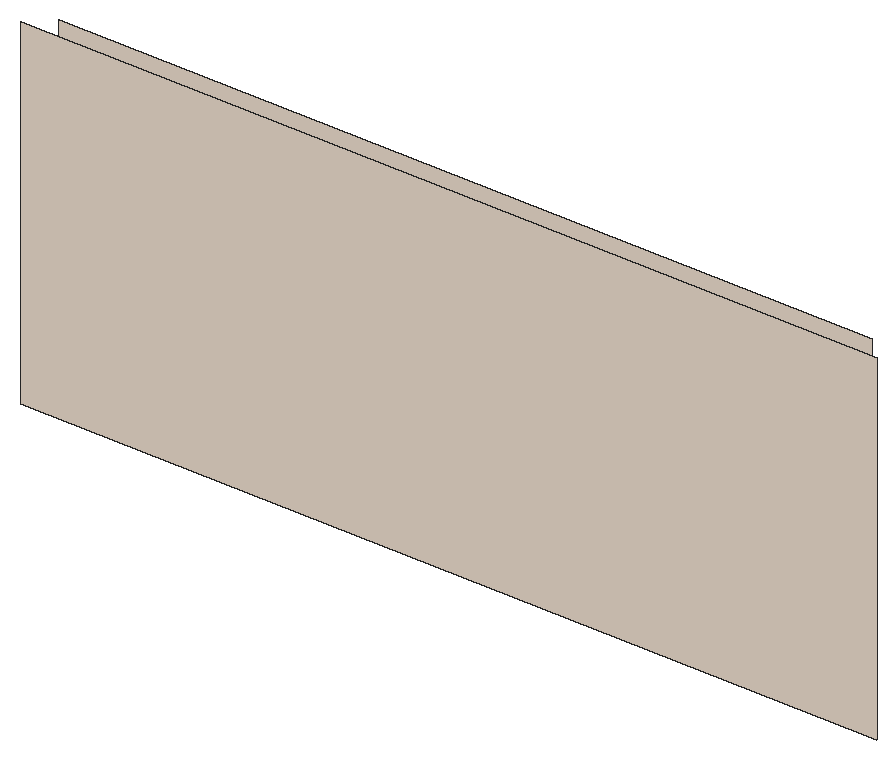
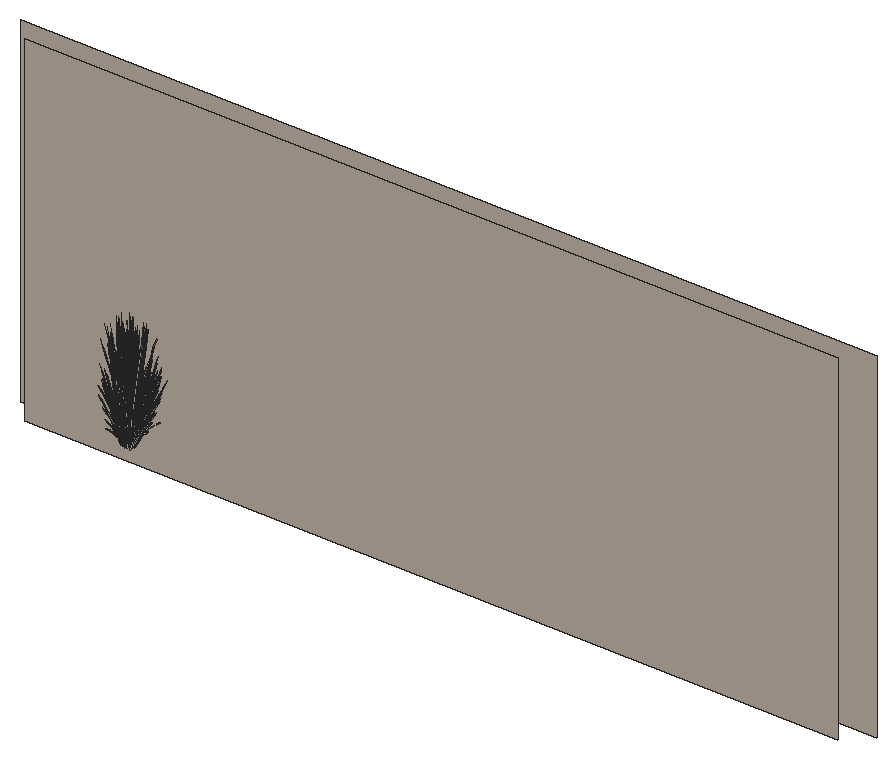
# SketchUp Ruby script. Lengths in inches.
U = 1.inch
M = Sketchup.active_model
def pt(a) = Geom::Point3d.new(a.map { |v| v * U })
def face(e, loops, mat)
  f = e.add_face(loops[0].map { |a| pt(a) })
  loops[1..].each { |l| e.add_face(l.map { |a| pt(a) }).erase! }
  f.material = f.back_material = mat if mat
  f
end
# faces: each face lists its corners as indices into pts; further lists are holes
def faces(e, pts, list, mat = nil) = list.each { |f| face(e, (f[0].is_a?(Array) ? f : [f]).map { |l| l.map { |i| pts[i] } }, mat) }
# xy, xz, yz: faces in a plane at the given z, y or x. An outline is a flat list of corners, or four numbers for a rectangle; further outlines are holes
def ring(l) = l.size == 4 ? [[l[0], l[1]], [l[2], l[1]], [l[2], l[3]], [l[0], l[3]]] : l.each_slice(2).to_a
def flat(e, list, mat, &to3) = list.each { |f| face(e, (f[0].is_a?(Array) ? f : [f]).map { |l| ring(l).map { |u, v| to3.(u, v) } }, mat) }
def xy(e, z, list, mat = nil) = flat(e, list, mat) { |x, y| [x, y, z] }
def xz(e, y, list, mat = nil) = flat(e, list, mat) { |x, z| [x, y, z] }
def yz(e, x, list, mat = nil) = flat(e, list, mat) { |y, z| [x, y, z] }
def lines(e, pts, list) = list.each { |a, b| e.add_line(pt(pts[a]), pt(pts[b])) }
# prism: a flat outline (further loops are holes) pulled along v
def prism(e, loops, v, mat = nil)
  f = face(e, loops, mat); d = Geom::Vector3d.new(v.map { |x| x * U })
  f.pushpull(f.normal.samedirection?(d) ? d.length : -d.length)
end
def box(e, o, s, mat = nil) = prism(e, [[o, [o[0] + s[0], o[1], o[2]], [o[0] + s[0], o[1] + s[1], o[2]], [o[0], o[1] + s[1], o[2]]]], [0, 0, s[2]], mat)
def at(x, y, z, deg = 0) = Geom::Transformation.translation(pt([x, y, z])) * Geom::Transformation.rotation(ORIGIN, Z_AXIS, deg.degrees)
def axes(o, x, y, z) = Geom::Transformation.new([*x, 0, *y, 0, *z, 0, *pt(o).to_a, 1])
def part(name) = M.definitions.add(name)
# library, detail: a bought-in or finely detailed component or shape, given as its bounding box
def library(name, o, s) = part(name).tap { |d| box(d.entities, o, s) }
def detail(e, o, s) = box(e.add_group.entities, o, s)
def put(e, d, t, mat = nil) = e.add_instance(d, t).tap { |i| i.material = mat if mat }
def group(e, t, mat = nil) = e.add_group.tap { |g| g.transformation = t; g.material = mat if mat }.entities
root = M.entities
M.materials.add("C01_Vanilla_Cream").color = [244, 228, 212]
M.materials.add("LightPink_Translucent").color = [144, 107, 117]
M.materials["LightPink_Translucent"].alpha = 0.75
c1 = part("blade")
p = [[2.15,0.21,22],[0,0.17,0],[0.09,0.45,0],[2.18,0.31,22],[2.29,0.31,22],[0.38,0.45,0],
  [2.48,0.24,33],[2.49,0.24,33],[2.48,0.22,33]]
faces(c1.entities,p,[[0,1,2,3],[4,5,2,3],[6,3,4,7],[8,0,3,6]])
c2 = part("seeds")
p = [[0.3,-0.1,1.38],[-0.01,-0.03,1.59],[-0.01,-0.03,0.03],[0.14,-0.07,-0.07],[0.29,-0.03,3],[0.15,0.01,3.11]]
faces(c2.entities,p,[[0,1,2,3],[1,0,4,5]],"LightPink_Translucent")
c3 = part("blade with seeds")
put(c3.entities,c1,at(0,0,0))
put(c3.entities,c2,axes([2.4,0.25,30.99],[1.5799,-0.05474,1.17369],[-0.12525,1.92788,0.29478],[-0.07173,-0.02425,1.56792]))
xz(root,0,[[0,450,360,594]],"C01_Vanilla_Cream")
xz(root,9,[[9,450,351,594]],"C01_Vanilla_Cream")
put(root,c3,axes([293.83,22.27,468.09],[0.23093,-0.01116,1.28532],[-0.15319,0.4836,0.10393],[-0.32909,-0.02991,0.54946]))
put(root,c3,axes([293.93,23.12,468.09],[0.19317,-0.10421,1.28532],[0.16263,0.48153,0.10393],[-0.30326,0.10883,0.54946]))
put(root,c3,axes([293.32,23.9375,467.125],[0.19348,0.04044,1.07251],[0.1247,0.41309,-0.23066],[-0.26282,0.07733,0.45856]))
put(root,c3,axes([295.04,22.62,467.6875],[0.15825,-0.07127,1.32798],[0.05457,0.4976,0.10393],[-0.34278,0.06603,0.47463]))
put(root,c3,axes([293.34,22.95,468.72],[-0.09091,0.06396,1.31208],[0.00773,0.46734,-0.2075],[-0.20839,0.06078,0.10523]))
put(root,c3,axes([294.52,21.82,468.92],[-0.55654,-0.01186,-0.53284],[0.03738,-0.49951,0.0643],[-0.23578,-0.05271,0.75375]))
put(root,c3,axes([294.07,21.94,467.125],[0.1087,0.13716,1.07251],[-0.25048,0.37284,-0.23066],[-0.25719,-0.08912,0.45856]))
put(root,c3,axes([293.63,22.68,468.58],[-0.46269,-0.13744,-0.2656],[0.13495,-0.40096,0.3429],[-0.18628,0.03677,0.65611]))
put(root,c3,axes([294.27,21.49,468.09],[0.2068,0.08488,1.28532],[-0.42797,0.35609,0.10393],[-0.26673,-0.16064,0.54946]))
put(root,c3,axes([292.33,23.42,468.71],[0.07105,0.01321,1.33037],[0.2198,0.43529,-0.12571],[-0.14545,0.11425,0.23543]))
put(root,c3,axes([293.94,22.89,468.69],[-0.15083,0.44814,-0.38324],[-0.51712,-0.15361,-0.29685],[-0.2082,0.04109,0.7333]))
put(root,c3,axes([294.34,21.92,468.69],[-0.40426,0.32635,-0.38324],[-0.35404,-0.34474,-0.29685],[-0.2054,-0.04965,0.7333]))
put(root,c3,axes([293.68,22.86,466.3],[0.01412,0.07764,1.32257],[-0.28464,0.40547,-0.20205],[-0.20218,-0.02044,0.22528]))
put(root,c3,axes([293.77,21,468.71],[0.04127,0.04917,1.33037],[-0.19898,0.44196,-0.12571],[-0.20151,0.0032,0.23543]))
put(root,c3,axes([292.92,24.8,467.26],[0.23202,-0.22328,0.86145],[0.09155,0.35348,0.63294],[-0.16768,0.06329,0.18974]))
put(root,c3,axes([294.23,20.71,468.72],[-0.11979,-0.00348,1.31208],[-0.38137,0.34775,-0.2075],[-0.20349,-0.07106,0.10523]))
put(root,c3,axes([293.73,22.63,468.73],[0.15729,-0.44921,0.36002],[0.51712,0.15361,0.29685],[-0.20336,0.027,0.74497]))
put(root,c3,axes([293.92,22.5,468.96],[0.28012,0.44611,-0.0912],[-0.49717,0.21923,-0.50621],[-0.20951,0.05886,0.76918]))
put(root,c3,axes([294.55,21.58,468.96],[-0.02981,0.50103,-0.0912],[-0.56442,-0.01369,-0.50621],[-0.21738,-0.0348,0.76918]))
put(root,c3,axes([294.1875,21.61,468.58],[-0.31678,-0.30846,-0.2656],[0.36171,-0.29199,0.3429],[-0.18378,-0.04443,0.65611]))
put(root,c3,axes([293.7,22.51,468.73],[-0.20448,-0.33592,0.04823],[0.37288,-0.16442,0.37966],[-0.16437,0.03244,0.57892]))
put(root,c3,axes([294.63,23.44,468.09],[0.13906,-0.15138,1.28532],[0.35111,0.40859,0.10393],[-0.24082,0.18608,0.54946]))
put(root,c3,axes([293.8,23.84,468.58],[-0.48462,0.07041,-0.2656],[-0.12797,-0.4025,0.3429],[-0.13888,0.10811,0.65611]))
put(root,c3,axes([293.53,25.03,466.3],[0.07468,0.04922,1.32257],[0.12663,0.45605,-0.20205],[-0.16551,0.09725,0.22528]))
put(root,c3,axes([293.43,22.35,467.26],[0.35544,-0.03525,0.86145],[-0.22547,0.31061,0.63294],[-0.17565,-0.04659,0.18974]))
put(root,c3,axes([293.86,23.75,468.73],[-0.13808,-0.45342,0.36002],[0.54163,-0.07869,0.29685],[-0.15963,0.10664,0.74497]))
put(root,c3,axes([294.14,21.5,469],[0.45978,-0.36358,0.40322],[0.39653,0.38611,0.33247],[-0.21571,-0.06707,0.83437]))
put(root,c3,axes([293.75,23.66,468.73],[-0.3822,-0.20719,0.04823],[0.22252,-0.29505,0.37966],[-0.12254,0.09539,0.57892]))
put(root,c3,axes([294.53,23.82,468.09],[0.10366,-0.16934,1.28532],[0.43488,0.35044,0.10393],[-0.19618,0.21841,0.54946]))
put(root,c3,axes([294.11,22.64,468.97],[0.46269,0.13744,0.2656],[-0.13495,0.40096,-0.3429],[-0.18628,0.03677,0.65611]))
put(root,c3,axes([294.2,23.89,468.69],[0.14302,0.44985,-0.38324],[-0.54163,0.07869,-0.29685],[-0.15522,0.12083,0.7333]))
put(root,c3,axes([294.35,21.49,468.73],[0.02803,-0.37463,0.04823],[0.42332,0.01027,0.37966],[-0.16216,-0.0392,0.57892]))
put(root,c3,axes([293.35,24.69,468.72],[-0.01384,0.09749,1.31208],[0.39274,0.33916,-0.2075],[-0.10282,0.16039,0.10523]))
put(root,c3,axes([295.55,23.5625,466.73],[-0.57914,-0.08077,-0.46765],[0.12221,-0.49823,-0.12274],[-0.17283,-0.06037,1.03225]))
put(root,c3,axes([295.65,20.85,469.25],[-0.37157,0.4723,-0.10215],[-0.5381,-0.2721,-0.56695],[-0.18705,-0.13344,0.86148]))
put(root,c3,axes([294.64,21.77,468.97],[0.31678,0.30846,0.2656],[-0.36171,0.29199,-0.3429],[-0.18378,-0.04443,0.65611]))
put(root,c3,axes([295.49,21.23,468.92],[-0.47473,-0.23813,-0.53284],[0.33738,-0.41728,0.0643],[-0.172,-0.14218,0.75375]))
put(root,c3,axes([295.27,21.24,468.69],[-0.54938,0.11711,-0.38324],[-0.0961,-0.44351,-0.29685],[-0.14756,-0.1271,0.7333]))
put(root,c3,axes([294.79,24.51,466.69],[-0.52105,-0.24633,-0.37238],[0.31144,-0.44171,0],[-0.11867,-0.0561,1.18128]))
put(root,c3,axes([294.56,20.84,466.3],[-0.05393,0.0649,1.32257],[-0.545,0.13993,-0.20205],[-0.13166,-0.12729,0.22528]))
put(root,c3,axes([293.94,23.5625,468.96],[0.515,0.27165,-0.0912],[-0.2967,0.3934,-0.50621],[-0.1455,0.13675,0.76918]))
put(root,c3,axes([295.1,24.8,466.96],[-0.34808,0.49367,0],[-0.58235,-0.27531,-0.38706],[-0.13264,-0.0627,1.22783]))
put(root,c3,axes([293.09,24.74,469.42],[0.49129,0.13151,-0.04866],[-0.15113,0.40475,-0.22062],[-0.08035,0.06145,0.72768]))
put(root,c3,axes([294.19,23.6,468.97],[0.48462,-0.07041,0.2656],[0.12797,0.4025,-0.3429],[-0.13888,0.10811,0.65611]))
put(root,c3,axes([294.47,25.52,467.125],[0.17569,-0.07772,1.07251],[0.43377,0.23434,-0.23066],[-0.12911,0.20277,0.45856]))
put(root,c3,axes([294.22,21.09,466.78],[-0.1606,0.40228,-0.02919],[-0.4943,-0.12375,-0.13237],[-0.07505,-0.0658,0.43661]))
put(root,c3,axes([295.51,19.72,468.71],[-0.01039,0.05905,1.33037],[-0.51226,0.21431,-0.12571],[-0.15074,-0.10955,0.23543]))
put(root,c3,axes([294.96,20.58,467.125],[-0.03371,0.16116,1.07251],[-0.49286,0.13491,-0.23066],[-0.11521,-0.20831,0.45856]))
put(root,c3,axes([295.12,21,468.09],[0.12726,0.15818,1.28532],[-0.58807,0.13317,0.10393],[-0.13291,-0.24832,0.54946]))
put(root,c3,axes([296.2,23.64,467.18],[-0.56211,0.32708,-0.21822],[-0.3738,-0.46216,-0.37502],[-0.13869,-0.04694,1.19781]))
put(root,c3,axes([294.65,24.67,468.73],[-0.39645,-0.33614,0.36002],[0.42102,-0.2899,0.29685],[-0.07313,0.15771,0.74497]))
put(root,c3,axes([295.32,20.91,468.58],[-0.08599,-0.39682,-0.2656],[0.49155,-0.10478,0.3429],[-0.13203,-0.11372,0.65611]))
put(root,c3,axes([293.95,22.92,466.96],[-0.69617,0,0],[0,-0.55062,-0.38706],[0,-0.12541,1.22783]))
put(root,c3,axes([294.93,24.32,466.7],[-0.13078,-0.42928,-0.23233],[0.51941,-0.1219,0.23233],[-0.10471,-0.0495,1.0423]))
put(root,c3,axes([294.5,24.64,468.73],[-0.45752,-0.02296,0.04823],[0.01254,-0.34663,0.37966],[-0.04787,0.13278,0.57892]))
put(root,c3,axes([294.65,24.77,468.58],[-0.3767,0.25939,-0.2656],[-0.3566,-0.29618,0.3429],[-0.05426,0.15048,0.65611]))
put(root,c3,axes([296.58,23.99,466.73],[-0.375,0.3703,-0.46765],[-0.46584,-0.33578,-0.12274],[-0.15027,0.09237,1.03225]))
put(root,c3,axes([295.62,21.24,468.97],[0.08599,0.39682,0.2656],[-0.49155,0.10478,-0.3429],[-0.13203,-0.11372,0.65611]))
put(root,c3,axes([293.31,25.69,468.71],[0.06316,-0.02974,1.33037],[0.52204,0.19785,-0.12571],[-0.01227,0.16473,0.23543]))
put(root,c3,axes([294.49,22.78,466.93],[-0.51786,0.4142,0.23067],[-0.51817,-0.40984,-0.27369],[-0.01808,-0.11762,1.23664]))
put(root,c3,axes([296.625,23.92,467.68],[0.48111,0.19866,1.13446],[-0.47133,0.42798,0.44862],[-0.21112,-0.25366,0.95105]))
put(root,c3,axes([294.79,20.32,467.26],[0.29042,0.17147,0.86145],[-0.42295,0.10307,0.63294],[-0.0905,-0.13178,0.18974]))
put(root,c3,axes([296.83,23.79,467.03],[-0.54364,-0.39653,-0.18894],[0.45745,-0.44527,0.41347],[-0.14639,0.04639,1.26162]))
put(root,c3,axes([295.85,23.4,466.84],[-0.33445,-0.41351,-0.33554],[0.50659,-0.29119,0.16149],[-0.10823,-0.05117,1.07733]))
put(root,c3,axes([294.9,24.5,469.19],[-0.01449,0.45571,-0.59145],[-0.61002,-0.03061,0.07138],[-0.06438,0.19306,0.83667]))
put(root,c3,axes([294.89,25.78,467.26],[-0.01441,-0.29294,0.86145],[0.36003,0.20894,0.63294],[-0.07081,0.13963,0.18974]))
put(root,c3,axes([295.39,20.77,469],[0.62019,-0.12663,0.40322],[0.10763,0.49673,0.33247],[-0.14586,-0.1464,0.83437]))
put(root,c3,axes([296.56,23.7,466.84],[-0.60457,0.03041,-0.33554],[-0.05467,-0.50484,0.16149],[-0.10823,0.05117,1.07733]))
put(root,c3,axes([295.54,20.88,468.73],[0.25304,-0.31296,0.04823],[0.36033,0.18221,0.37966],[-0.11649,-0.10034,0.57892]))
put(root,c3,axes([295.4,24.55,467.04],[0.52105,0.24633,0.37238],[-0.31144,0.44171,0],[-0.11867,-0.0561,1.18128]))
put(root,c3,axes([294.7,25.14,467.7],[0.01223,-0.25433,1.15759],[0.55017,0.13434,0.15997],[-0.04767,0.27105,0.54661]))
put(root,c3,axes([295.9,23.64,467.01],[0.14756,-0.58378,-0.17572],[0.69966,0.10176,0.38453],[-0.12225,-0.08062,1.1733]))
put(root,c3,axes([296.15,23.78,467.14],[-0.1074,0.43968,0.1086],[-0.52474,-0.07632,-0.3101],[-0.0955,-0.04515,0.95058]))
put(root,c3,axes([296.09,19.95,468.72],[-0.08515,-0.06907,1.31208],[-0.56828,0.04379,-0.2075],[-0.0907,-0.16522,0.10523]))
put(root,c3,axes([297.19,25,466.69],[-0.52105,0.24633,-0.37238],[-0.31144,-0.44171,0],[-0.11867,0.0561,1.18128]))
put(root,c3,axes([294.11,22.55,466.69],[0,-0.49266,-0.37238],[0.62289,0,0],[0,-0.11221,1.18128]))
put(root,c3,axes([294.375,23.01,467.04],[0,0.49266,0.37238],[-0.62289,0,0],[0,-0.11221,1.18128]))
put(root,c3,axes([297.23,24.87,466.83],[-0.34375,-0.4954,-0.03857],[0.58235,-0.27531,0.38706],[-0.1435,0.04717,1.22723]))
put(root,c3,axes([295.02,24.65,468.94],[0.39855,0.33102,-0.4254],[-0.42102,0.2899,-0.32951],[-0.06064,0.16819,0.81396]))
put(root,c3,axes([297.07,24.81,466.7],[-0.51941,-0.1219,-0.23233],[0.13078,-0.42928,0.23233],[-0.10471,0.0495,1.0423]))
put(root,c3,axes([294.85,24.4,468.97],[0.3767,-0.25939,0.2656],[0.3566,0.29618,-0.3429],[-0.05426,0.15048,0.65611]))
put(root,c3,axes([295.74,23.12,467.18],[-0.62699,-0.23507,-0.21822],[0.3019,-0.49615,-0.37502],[-0.0197,-0.12182,1.19781]))
put(root,c3,axes([297.37,22.97,467.3125],[-0.01521,-0.46386,1.05954],[0.68831,0.12024,0.44862],[-0.1628,0.25382,1.00012]))
put(root,c3,axes([294.61,24.47,469.23],[0.61188,0.02441,-0.10123],[-0.01672,0.46217,-0.56189],[-0.0425,0.178,0.85379]))
put(root,c3,axes([294.59,25.15,467.3],[0.50577,-0.08724,0.04881],[0.11627,0.35148,-0.64728],[-0.03206,0.17792,0.5802]))
put(root,c3,axes([296.98,23.57,467.18],[0.06488,0.56215,-0.21822],[-0.6757,0.03399,-0.37502],[-0.11898,0.07488,1.19781]))
put(root,c3,axes([295.46,22.62,466.75],[-0.22864,-0.5052,-0.52377],[0.65862,-0.18195,-0.13747],[-0.02527,-0.17107,1.15612]))
put(root,c3,axes([296.95,21.02,468.96],[-0.54481,0.22937,-0.0912],[-0.26773,-0.4071,-0.50621],[-0.07188,-0.17155,0.76918]))
put(root,c3,axes([296.49,21.04,468.69],[-0.54728,-0.1235,-0.38324],[0.18759,-0.42344,-0.29685],[-0.05018,-0.17048,0.7333]))
put(root,c3,axes([295.48,24.17,468.09],[-0.01363,-0.18909,1.28532],[0.5906,0.12544,0.10393],[-0.03653,0.26947,0.54946]))
put(root,c3,axes([294.375,22.5625,466.7],[0.38863,-0.30738,-0.23233],[0.38863,0.30738,0.23233],[0,-0.09901,1.0423]))
put(root,c3,axes([296.13,20.57,466.78],[-0.38473,0.28263,-0.02919],[-0.35252,-0.30954,-0.13237],[-0.02482,-0.08771,0.43661]))
put(root,c3,axes([295.98,23.36,466.95],[0.70367,0.1038,0.34316],[-0.1432,0.58624,0.13466],[-0.10283,-0.05661,1.19142]))
put(root,c3,axes([295.79,23.25,467.22],[-0.27012,0.44393,0.33554],[-0.56127,-0.21365,-0.16149],[0,-0.10233,1.07733]))
put(root,c3,axes([296.6875,21.12,468.92],[-0.26572,-0.40059,-0.53284],[0.54698,-0.22325,0.0643],[-0.06214,-0.19355,0.75375]))
put(root,c3,axes([295.6,24.3,467.04],[0.59825,-0.13076,0.13232],[0.14773,0.48663,0.26315],[-0.05336,-0.0709,1.20305]))
put(root,c3,axes([296.37,24.375,466.83],[-0.56127,-0.22118,0],[0.27012,-0.45959,0],[0,0,1.2203]))
put(root,c3,axes([296.79,21.17,468.97],[-0.16784,0.37886,0.2656],[-0.48968,-0.1105,-0.3429],[-0.0449,-0.15254,0.65611]))
put(root,c3,axes([297.67,24.93,466.96],[0.34808,0.49367,0],[-0.58235,0.27531,-0.38706],[-0.13264,0.0627,1.22783]))
put(root,c3,axes([295.9,25.14,468.98],[-0.54859,-0.1288,0.39962],[0.18759,-0.42344,0.32951],[0.03297,0.16652,0.82692]))
put(root,c3,axes([295.75,25.17,468.73],[-0.41024,0.16744,0.04823],[-0.2008,-0.30532,0.37966],[0.03962,0.13459,0.57892]))
put(root,c3,axes([297.38,24.32,467.04],[0.16083,-0.48962,0.13232],[0.58854,0.13856,0.26315],[-0.10167,0.00238,1.20305]))
put(root,c3,axes([297.11,23.67,467.14],[0.41131,0.296,0.1086],[-0.34309,0.33395,-0.3101],[-0.0955,0.04515,0.95058]))
put(root,c3,axes([296.96,23.31,466.9],[-0.51786,-0.42404,-0.04598],[0.51817,-0.4243,0],[-0.01808,-0.01481,1.31678]))
put(root,c3,axes([297.1,23.46,467.22],[0.60457,-0.03041,0.33554],[0.05467,0.50484,-0.16149],[-0.10823,0.05117,1.07733]))
put(root,c3,axes([297.24,24.62,466.93],[0.697,0.16013,0.23067],[-0.17437,0.57237,-0.27369],[-0.11536,0.07164,1.23664]))
put(root,c3,axes([296.23,20.23,466.3],[-0.09338,0.01775,1.32257],[-0.51641,-0.1998,-0.20205],[0.00867,-0.16666,0.22528]))
put(root,c3,axes([297.54,24.59,467.04],[0.52105,-0.24633,0.37238],[0.31144,0.44171,0],[-0.11867,0.0561,1.18128]))
put(root,c3,axes([296.74,20.78,468.58],[0.16784,-0.37886,-0.2656],[0.48968,0.1105,0.3429],[-0.0449,-0.15254,0.65611]))
put(root,c3,axes([295.92,22.82,466.95],[0.24206,0.5509,0.34316],[-0.69162,0.19157,0.13466],[0.00845,-0.10123,1.19142]))
put(root,c3,axes([295.8,22.75,466.84],[0.27012,-0.44393,-0.33554],[0.56127,0.21365,0.16149],[0,-0.10233,1.07733]))
put(root,c3,axes([296.5,24.18,466.83],[-0.18165,-0.42474,0],[0.51872,-0.14874,0],[0,0,1.15778]))
put(root,c3,axes([295.84,25.08,466.3],[0.0901,-0.02681,1.32257],[0.54199,0.14755,-0.20205],[0.01585,0.1663,0.22528]))
put(root,c3,axes([295.96,25.23,468.58],[-0.16784,0.37886,-0.2656],[-0.48968,-0.1105,0.3429],[0.0449,0.15254,0.65611]))
put(root,c3,axes([297.23,23.35,466.84],[-0.27012,0.44393,-0.33554],[-0.56127,-0.21365,0.16149],[0,0.10233,1.07733]))
put(root,c3,axes([296.94,20.83,468.73],[0.41024,-0.16744,0.04823],[0.2008,0.30532,0.37966],[-0.03962,-0.13459,0.57892]))
put(root,c3,axes([295.61,25.9,468.72],[0.07057,0.07933,1.31208],[0.56952,0.03117,-0.2075],[0.05727,0.17496,0.10523]))
put(root,c3,axes([298.3,23.07,467.04],[-0.43742,-0.35886,0.13232],[0.44081,-0.34807,0.26315],[-0.04831,0.07329,1.20305]))
put(root,c3,axes([296.79,22.87,466.84],[0,-0.57005,0],[0.69617,0,0],[0,0,1.34592]))
put(root,c3,axes([296.8,20.86,468.73],[0.54859,0.1288,0.36002],[-0.18759,0.42344,0.29685],[-0.03297,-0.16652,0.74497]))
put(root,c3,axes([296.14,22.97,467.01],[0.6273,0.23878,0.18048],[-0.3019,0.49615,0.37502],[0,-0.11437,1.20407]))
put(root,c3,axes([297.14,23.1,466.9],[0,0.56976,-0.04228],[-0.69617,0,0],[0,0.01791,1.34526]))
put(root,c3,axes([295.9375,22.64,467.22],[-0.60457,0.03041,0.33554],[-0.05467,-0.50484,-0.16149],[0.10823,-0.05117,1.07733]))
put(root,c3,axes([295.9,24.83,468.97],[0.16784,-0.37886,0.2656],[0.48968,0.1105,-0.3429],[0.0449,0.15254,0.65611]))
put(root,c3,axes([295.66,21.77,467.04],[-0.16083,0.48962,0.13232],[-0.58854,-0.13856,0.26315],[0.10167,-0.00238,1.20305]))
put(root,c3,axes([296.8,24.2,466.9],[0.24206,0.56598,-0.04509],[-0.69162,0.19832,0],[0.00845,0.01976,1.2913]))
put(root,c3,axes([295.37,21.17,466.96],[-0.34808,-0.49367,0],[0.58235,-0.27531,-0.38706],[0.13264,-0.0627,1.22783]))
put(root,c3,axes([296.01,24.89,468.92],[0.26572,0.40059,-0.53284],[-0.54698,0.22325,0.0643],[0.06214,0.19355,0.75375]))
put(root,c3,axes([298.8,23.46,466.83],[-0.69582,-0.00394,-0.03732],[0,-0.55062,0.37457],[-0.02187,0.12535,1.18764]))
put(root,c3,axes([297.4375,21.8,467.04],[-0.59825,0.13076,0.13232],[-0.14773,-0.48663,0.26315],[0.05336,0.0709,1.20305]))
put(root,c3,axes([296.82,19.98,467.26],[0.07142,0.28728,0.86145],[-0.3962,-0.15911,0.63294],[0.04263,-0.1471,0.18974]))
put(root,c3,axes([296.5625,26.18,469.42],[0.38473,-0.28263,-0.04866],[0.35252,0.30954,-0.22062],[0.02482,0.08771,0.72768]))
put(root,c3,axes([296.46,22.51,466.95],[-0.46162,0.4471,0.34316],[-0.54842,-0.39467,0.13466],[0.11129,-0.04462,1.19142]))
put(root,c3,axes([297.25,23.21,466.84],[0.38863,0.31822,0],[-0.38863,0.31822,0],[0,0,1.2695]))
put(root,c3,axes([297.24,22.84,467.22],[0.27012,-0.44393,0.33554],[0.56127,0.21365,-0.16149],[0,0.10233,1.07733]))
put(root,c3,axes([297.01,24.38,466.83],[0.56127,0.22118,0],[-0.27012,0.45959,0],[0,0,1.31215]))
put(root,c3,axes([296.21,24.97,468.69],[0.54728,0.1235,-0.38324],[-0.18759,0.42344,-0.29685],[0.05018,0.17048,0.7333]))
put(root,c3,axes([295.74,24.99,468.96],[0.54481,-0.22937,-0.0912],[0.26773,0.4071,-0.50621],[0.07188,0.17155,0.76918]))
put(root,c3,axes([297.06,22.74,466.97],[-0.70367,-0.1038,0.36899],[0.1432,-0.58624,0.1448],[0.10283,0.05661,1.2811]))
put(root,c3,axes([298.52,20.44,468.71],[-0.05654,0.03763,1.33037],[-0.55396,-0.12696,-0.12571],[-0.02005,-0.16422,0.23543]))
put(root,c3,axes([298.09,21.53,468.96],[-0.61188,-0.02441,-0.0912],[0.01672,-0.46217,-0.50621],[0.0425,-0.178,0.76918]))
put(root,c3,axes([298.66,23.54,466.7],[-0.38863,0.30738,-0.23233],[-0.38863,-0.30738,0.23233],[0,0.09901,1.0423]))
put(root,c3,axes([297.55,23.48,466.75],[0.20414,0.45107,-0.51909],[-0.58805,0.16245,-0.13624],[0.02256,0.15274,1.1458]))
put(root,c3,axes([297.26,23,466.84],[0.62289,0,0],[0,0.51004,0],[0,0,1.33805]))
put(root,c3,axes([297.85,21.6,468.97],[-0.3767,0.25939,0.2656],[-0.3566,-0.29618,-0.3429],[0.05426,-0.15048,0.65611]))
put(root,c3,axes([296.66,22.43,467.22],[-0.33445,-0.41351,0.33554],[0.50659,-0.29119,-0.16149],[0.10823,0.05117,1.07733]))
put(root,c3,axes([296.05,22.53,467.18],[-0.06488,-0.56215,-0.21822],[0.6757,-0.03399,-0.37502],[0.11898,-0.07488,1.19781]))
put(root,c3,axes([297.47,22.94,467.14],[0.51872,-0.14368,0.1086],[0.18165,0.41027,-0.3101],[0,0.09029,0.95058]))
put(root,c3,axes([297.67,21.36,468.69],[-0.39855,-0.33102,-0.38324],[0.42102,-0.2899,-0.29685],[0.06064,-0.16819,0.7333]))
put(root,c3,axes([297.3,22.98,467.18],[0.62699,0.23507,-0.21822],[-0.3019,0.49615,-0.37502],[0.0197,0.12182,1.19781]))
put(root,c3,axes([295.96,21.29,466.7],[0.51941,0.1219,-0.23233],[-0.13078,0.42928,0.23233],[0.10471,-0.0495,1.0423]))
put(root,c3,axes([297.41,20.77,467.125],[-0.15825,0.09972,1.07251],[-0.47395,-0.17454,-0.23066],[0.08785,-0.21706,0.45856]))
put(root,c3,axes([298.66,23.09,467.04],[0,-0.49266,0.37238],[0.62289,0,0],[0,0.11221,1.18128]))
put(root,c3,axes([298.93,23.55,466.69],[0,0.49266,-0.37238],[-0.62289,0,0],[0,0.11221,1.18128]))
put(root,c3,axes([297.26,25.04,468.73],[-0.55374,0.11306,0.36002],[-0.0961,-0.44351,0.29685],[0.13023,0.13071,0.74497]))
put(root,c3,axes([295.84,21.09,466.69],[0.52105,-0.24633,-0.37238],[0.31144,0.44171,0],[0.11867,-0.0561,1.18128]))
put(root,c3,axes([297.16,25.125,468.73],[-0.25304,0.31296,0.04823],[-0.36033,-0.18221,0.37966],[0.11649,0.10034,0.57892]))
put(root,c3,axes([296.52,24.1,468.09],[-0.12726,-0.15818,1.28532],[0.58807,-0.13317,0.10393],[0.13291,0.24832,0.54946]))
put(root,c3,axes([296.88,22.32,467.14],[0.1074,-0.43968,0.1086],[0.52474,0.07632,-0.3101],[0.0955,0.04515,0.95058]))
put(root,c3,axes([297.63,21.55,467.04],[-0.52105,-0.24633,0.37238],[0.31144,-0.44171,0],[0.11867,0.0561,1.18128]))
put(root,c3,axes([297.79,21.51,468.92],[0.01449,-0.45571,-0.53284],[0.61002,0.03061,0.0643],[0.06438,-0.19306,0.75375]))
put(root,c3,axes([297.18,24.125,466.82],[0.5845,-0.16716,-0.14398],[0.20539,0.48152,0.00006],[0.06452,-0.01848,1.30423]))
put(root,c3,axes([297.08,24.77,468.97],[-0.08599,-0.39682,0.2656],[0.49155,-0.10478,-0.3429],[0.13203,0.11372,0.65611]))
put(root,c3,axes([297.1875,22.69,466.84],[0.33445,0.41351,-0.33554],[-0.50659,0.29119,0.16149],[0.10823,0.05117,1.07733]))
put(root,c3,axes([297.41,22.48,468.54],[-0.48108,-0.25598,1.03712],[0.50798,-0.39855,0.44749],[0.15521,0.24018,1.00248]))
put(root,c3,axes([298.04,21.23,468.58],[0.3767,-0.25939,-0.2656],[0.3566,0.29618,0.3429],[0.05426,-0.15048,0.65611]))
put(root,c3,axes([296.6,25.32,468.71],[0.00165,-0.05965,1.33037],[0.47711,-0.26315,-0.12571],[0.16572,0.09393,0.23543]))
put(root,c3,axes([298.1875,21.37,468.73],[0.45752,0.02296,0.04823],[-0.01254,0.34663,0.37966],[0.04787,-0.13278,0.57892]))
put(root,c3,axes([298.13,24.57,467.26],[-0.31347,-0.14166,0.86145],[0.40476,-0.14393,0.63294],[0.10917,0.12192,0.18974]))
put(root,c3,axes([297.02,24.42,467.125],[0.00982,-0.16331,1.07251],[0.4695,-0.18242,-0.23066],[0.14493,0.19547,0.45856]))
put(root,c3,axes([298.64,20.8,468.72],[-0.00537,-0.09805,1.31208],[-0.45391,-0.28338,-0.2075],[0.07018,-0.17178,0.10523]))
put(root,c3,axes([296.46,22.1,466.73],[0.375,-0.3703,-0.46765],[0.46584,0.33578,-0.12274],[0.15027,-0.09237,1.03225]))
put(root,c3,axes([298.04,21.33,468.73],[0.39645,0.33614,0.36002],[-0.42102,0.2899,0.29685],[0.07313,-0.15771,0.74497]))
put(root,c3,axes([298.1,21.77,466.7],[0.13078,0.42928,-0.23233],[-0.51941,0.1219,0.23233],[0.10471,0.0495,1.0423]))
put(root,c3,axes([299.08,23.17,466.96],[0.69617,0,0],[0,0.55062,-0.38706],[0,0.12541,1.22783]))
put(root,c3,axes([296.83,22.46,467.18],[0.56211,-0.32708,-0.21822],[0.3738,0.46216,-0.37502],[0.13869,0.04694,1.19781]))
put(root,c3,axes([298.18,25.21,467.18],[-0.35702,-0.01545,0.78795],[0.23577,-0.32816,0.43504],[0.14104,0.11659,0.61808]))
put(root,c3,axes([298.5,22.4,468.97],[-0.48462,0.07041,0.2656],[-0.12797,-0.4025,-0.3429],[0.13888,-0.10811,0.65611]))
put(root,c3,axes([297.11,21.28,468.09],[-0.10366,0.16934,1.28532],[-0.43488,-0.35044,0.10393],[0.19618,-0.21841,0.54946]))
put(root,c3,axes([297.03,24.97,468.96],[0.33176,-0.4217,-0.0912],[0.48044,0.24295,-0.50621],[0.16701,0.11914,0.76918]))
put(root,c3,axes([295.41,22.17,466.375],[-0.548,0.19724,0.96696],[-0.17442,-0.56594,0.37572],[0.3365,0.00941,1.09981]))
put(root,c3,axes([298.75,22.44,468.96],[-0.515,-0.27165,-0.0912],[0.2967,-0.3934,-0.50621],[0.1455,-0.13675,0.76918]))
